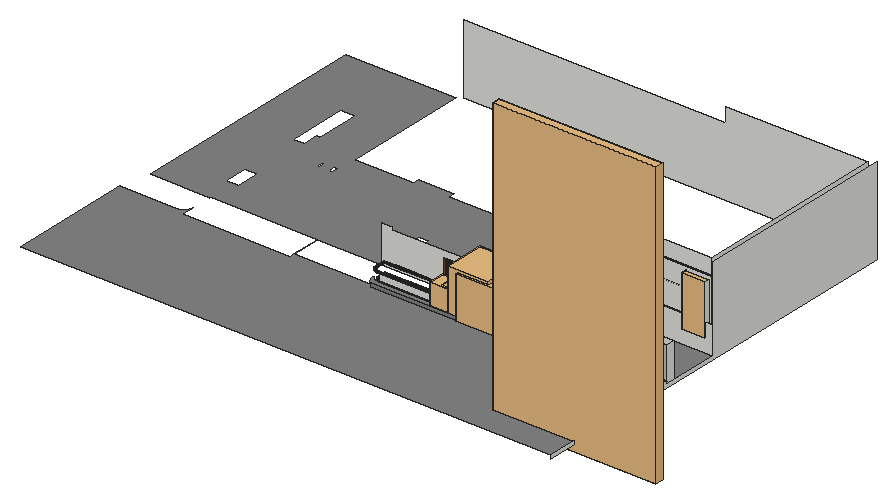
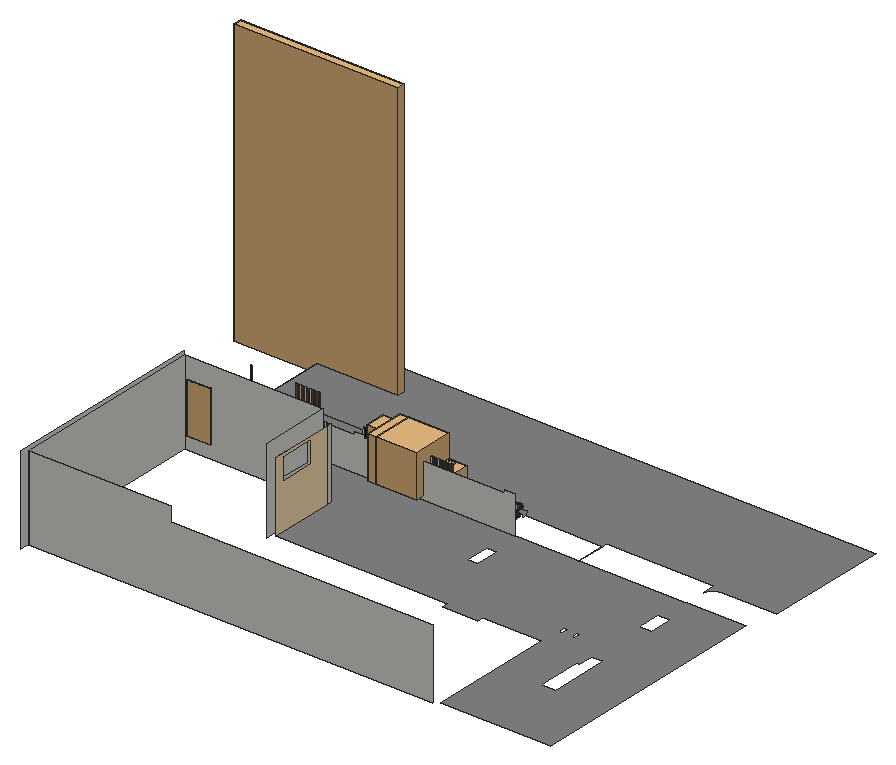
# SketchUp Ruby script. Lengths in inches.
U = 1.inch
M = Sketchup.active_model
def pt(a) = Geom::Point3d.new(a.map { |v| v * U })
def face(e, loops, mat)
  f = e.add_face(loops[0].map { |a| pt(a) })
  loops[1..].each { |l| e.add_face(l.map { |a| pt(a) }).erase! }
  f.material = f.back_material = mat if mat
  f
end
# faces: each face lists its corners as indices into pts; further lists are holes
def faces(e, pts, list, mat = nil) = list.each { |f| face(e, (f[0].is_a?(Array) ? f : [f]).map { |l| l.map { |i| pts[i] } }, mat) }
# xy, xz, yz: faces in a plane at the given z, y or x. An outline is a flat list of corners, or four numbers for a rectangle; further outlines are holes
def ring(l) = l.size == 4 ? [[l[0], l[1]], [l[2], l[1]], [l[2], l[3]], [l[0], l[3]]] : l.each_slice(2).to_a
def flat(e, list, mat, &to3) = list.each { |f| face(e, (f[0].is_a?(Array) ? f : [f]).map { |l| ring(l).map { |u, v| to3.(u, v) } }, mat) }
def xy(e, z, list, mat = nil) = flat(e, list, mat) { |x, y| [x, y, z] }
def xz(e, y, list, mat = nil) = flat(e, list, mat) { |x, z| [x, y, z] }
def yz(e, x, list, mat = nil) = flat(e, list, mat) { |y, z| [x, y, z] }
def lines(e, pts, list) = list.each { |a, b| e.add_line(pt(pts[a]), pt(pts[b])) }
# prism: a flat outline (further loops are holes) pulled along v
def prism(e, loops, v, mat = nil)
  f = face(e, loops, mat); d = Geom::Vector3d.new(v.map { |x| x * U })
  f.pushpull(f.normal.samedirection?(d) ? d.length : -d.length)
end
def box(e, o, s, mat = nil) = prism(e, [[o, [o[0] + s[0], o[1], o[2]], [o[0] + s[0], o[1] + s[1], o[2]], [o[0], o[1] + s[1], o[2]]]], [0, 0, s[2]], mat)
def at(x, y, z, deg = 0) = Geom::Transformation.translation(pt([x, y, z])) * Geom::Transformation.rotation(ORIGIN, Z_AXIS, deg.degrees)
def axes(o, x, y, z) = Geom::Transformation.new([*x, 0, *y, 0, *z, 0, *pt(o).to_a, 1])
def part(name) = M.definitions.add(name)
# library, detail: a bought-in or finely detailed component or shape, given as its bounding box
def library(name, o, s) = part(name).tap { |d| box(d.entities, o, s) }
def detail(e, o, s) = box(e.add_group.entities, o, s)
def put(e, d, t, mat = nil) = e.add_instance(d, t).tap { |i| i.material = mat if mat }
def group(e, t, mat = nil) = e.add_group.tap { |g| g.transformation = t; g.material = mat if mat }.entities
root = M.entities
M.materials.add("[0032_Moccasin]").color = [255, 228, 181]
M.materials.add("[0043_SaddleBrown]").color = [139, 69, 19]
M.materials.add("[0099_LightSteelBlue]").color = [82, 92, 104]
M.materials.add("[0131_Silver]").color = [192, 192, 192]
M.materials.add("[0136_Charcoal]").color = [35, 35, 35]
M.materials.add("[0137_Black]").color = [0, 0, 0]
M.materials.add("[Tile Grey]").color = [132, 132, 132]
M.materials.add("[Wood Veneer 01]").color = [120, 70, 37]
c1 = library("Potted plant on stand",[0,0,0],[37.88,32.09,49.42])
c2 = library("Pot+Plant",[-20.81,-17.08,-0.03],[39.86,39.43,41.33])
c3 = library("Agrupar\#180",[0,0,0],[49.83,35.16,80.22])
c4 = library("SPOT-EXTERIEUR",[0,-1.85,-3.93],[5.55,3.7,7.99])
c5 = library("A$C06767DEF\#1",[-8.3,1.21,0],[7.09,7.09,5.51])
c6 = library("door (1)",[38.93,25.48,0],[40,9.94,82.68])
c7 = library("Group\#87",[0,0,0],[185.03,8.78,321.45])
xy(root,6.6875,[[0,84.05,912.4375,84.05,912.4375,290.83,888.15,290.83,885.82,291.01,883.54,291.5625,881.37,292.46,879.37,293.68,877.59,295.2,876.0625,296.98,874.84,298.97,873.93,301.14,873.38,303.41,873.19,305.75,873.37,308.09,873.91,310.37,873.91,337.06,765.78,337.06,765.78,310.37,766.04,308.49,766.06,306.58,765.82,304.7,765.34,302.86,764.63,301.1,763.69,299.44,762.55,297.93,761.22,296.57,759.72,295.4,758.08,294.43,756.33,293.69,754.5,293.18,435,293.18,433.82,294.29,432.72,295.48,431.71,296.75,430.8,298.09,298.96,298.09,298.96,349.54,298.71,289.39,114.03,290.125,114.12,311.98,113.83,309.89,113.25,307.79,112.375,305.79,111.24,303.93,109.87,302.23,108.27,300.74,106.49,299.49,104.55,298.48,102.5,297.75,100.36,297.31,98.1875,297.16,0,297.16],[[12.79,349.54,114.27,349.54,114.27,350.28,298.96,349.54,912.4375,349.54,912.4375,431.86,798.1,431.86,798.1,432.24,795.91,432.24,795.91,431.86,720.28,431.86,720.28,432.24,713.72,432.24,713.72,433.11,711.84,433.11,711.84,432.24,705.28,432.24,705.28,433.11,703.41,433.11,703.41,432.17,696.84,432.17,696.84,433.11,694.97,433.11,694.97,432.17,688.41,432.17,688.41,433.11,686.53,433.11,686.53,432.17,679.97,432.17,679.97,433.11,677.84,433.11,677.84,432.17,671.28,432.17,671.28,433.11,669.16,433.11,669.16,432.17,666.61,432.17,666.61,431.86,660.05,431.86,660.05,551.1875,363.88,551.1875,363.88,562.07,303.76,562.07,303.76,551.1875,201.625,551.1875,201.625,768.3,12.79,768.3],[101.6875,542.92,101.6875,646.79,126.375,646.79,126.375,569.92,121.5,569.92,121.5,542.92],[101.6875,397.92,124.125,440.22],[400.76,397.92,418.84,440.22],[192.11,506.17,199.48,517.35],[171.55,506.17,177.8,517.35]]],"[Tile Grey]")
xy(root,11.9375,[[441.01,305.48,658.06,305.48,658.75,305.67,659.73,306.04,660.67,306.5,661.57,307.05,662.41,307.67,663.2,308.36,663.91,309.125,664.56,309.95,665.13,310.83,665.62,311.76,666.02,312.73,666.21,313.36,666.21,328.82,642.23,328.82,642.23,329,479.46,329,479.46,328.94,475.34,328.94,475.34,328.88,464.85,328.88,464.85,328.94,452.48,328.94,452.48,329,430.83,329,430.83,311.3,430.98,311.03,431.59,310.14,432.28,309.31,433.05,308.54,433.88,307.85,434.77,307.24,435.71,306.71,436.7,306.27,437.73,305.93,438.78,305.68,439.85,305.53]],"[0136_Charcoal]")
xy(root,11.9375,[[888.15,290.83,912.4375,290.83,912.4375,333.31,873.91,333.31,873.91,310.37,873.37,308.09,873.19,305.75,873.38,303.41,873.93,301.14,874.84,298.97,876.0625,296.98,877.59,295.2,879.37,293.68,881.37,292.46,883.54,291.5625,885.82,291.01],[435,293.18,754.5,293.18,756.33,293.69,758.08,294.43,759.72,295.4,761.22,296.57,762.55,297.93,763.69,299.44,764.63,301.1,765.34,302.86,765.82,304.7,766.06,306.58,766.04,308.49,765.78,310.37,765.78,333.31,683.875,333.31,683.875,331.81,669.83,331.81,669.83,312.81,669.42,311.49,668.89,310.22,668.25,309,667.51,307.85,666.66,306.77,665.71,305.77,664.6875,304.85,663.58,304.04,662.4,303.33,661.16,302.72,659.88,302.23,658.55,301.86,440.93,301.86,439.52,301.93,438.11,302.125,436.74,302.45,435.39,302.9,434.1,303.47,432.86,304.16,431.7,304.96,430.61,305.87,429.61,306.87,428.7,307.96,427.91,309.13,427.22,310.37,427.28,308.75,427.45,307.14,427.73,305.54,428.13,303.97,428.64,302.43,429.25,300.94,429.97,299.48,430.8,298.09,431.71,296.75,432.72,295.48,433.82,294.29]],"[Tile Grey]")
xy(root,17.45,[[765.78,337.06,873.91,337.87]])
xy(root,18.14,[[765.78,337.06,873.91,337.87]])
xy(root,26,[[[440.93,301.86,658.55,301.86,659.88,302.23,661.16,302.72,662.4,303.33,663.58,304.04,664.6875,304.85,665.71,305.77,666.66,306.77,667.51,307.85,668.25,309,668.89,310.22,669.42,311.49,669.83,312.81,669.83,333.31,669.72,333.31,669.72,332.43,666.47,332.43,666.47,333.31,665.6,333.31,665.6,332.43,662.34,332.43,662.34,333.31,661.47,333.31,661.47,332.43,658.22,332.43,658.22,333.31,657.35,333.31,657.35,332.43,654.09,332.43,654.09,333.31,653.22,333.31,653.22,332.43,649.97,332.43,649.97,333.31,649.1,333.31,649.1,332.43,645.84,332.43,645.84,333.31,644.97,333.31,644.97,332.62,641.72,332.62,641.72,333.31,640.85,333.31,640.85,332.62,637.59,332.62,637.59,333.31,636.72,333.31,636.72,332.62,633.47,332.62,633.47,333.31,632.6,333.31,632.6,332.62,629.34,332.62,629.34,333.31,628.47,333.31,628.47,332.62,625.22,332.62,625.22,333.31,624.35,333.31,624.35,332.62,621.09,332.62,621.09,333.31,620.22,333.31,620.22,332.62,616.97,332.62,616.97,333.31,616.1,333.31,616.1,332.62,612.84,332.62,612.84,333.31,611.97,333.31,611.97,332.62,608.72,332.62,608.72,333.31,607.85,333.31,607.85,332.62,604.59,332.62,604.59,333.31,603.72,333.31,603.72,332.62,600.47,332.62,600.47,333.31,599.6,333.31,599.6,332.62,596.34,332.62,596.34,333.31,595.47,333.31,595.47,332.62,592.22,332.62,592.22,333.31,591.35,333.31,591.35,332.62,588.09,332.62,588.09,333.31,587.22,333.31,587.22,332.62,583.97,332.62,583.97,333.31,583.1,333.31,583.1,332.62,579.84,332.62,579.84,333.31,578.97,333.31,578.97,332.62,575.72,332.62,575.72,333.31,574.85,333.31,574.85,332.62,571.59,332.62,571.59,333.31,570.72,333.31,570.72,332.62,567.47,332.62,567.47,333.31,566.6,333.31,566.6,332.62,563.34,332.62,563.34,333.31,562.47,333.31,562.47,332.62,559.22,332.62,559.22,333.31,558.35,333.31,558.35,332.62,555.09,332.62,555.09,333.31,554.22,333.31,554.22,332.62,550.97,332.62,550.97,333.31,550.1,333.31,550.1,332.62,546.84,332.62,546.84,333.31,545.97,333.31,545.97,332.62,542.72,332.62,542.72,333.31,541.85,333.31,541.85,332.62,538.59,332.62,538.59,333.31,537.72,333.31,537.72,332.62,534.47,332.62,534.47,333.31,533.6,333.31,533.6,332.62,530.34,332.62,530.34,333.31,529.47,333.31,529.47,332.62,526.22,332.62,526.22,333.31,525.35,333.31,525.35,332.62,522.09,332.62,522.09,333.31,521.22,333.31,521.22,332.62,517.97,332.62,517.97,333.31,517.1,333.31,517.1,332.62,513.84,332.62,513.84,333.31,512.97,333.31,512.97,332.62,509.72,332.62,509.72,333.31,508.85,333.31,508.85,332.62,505.59,332.62,505.59,333.31,504.72,333.31,504.72,332.62,501.47,332.62,501.47,333.31,500.6,333.31,500.6,332.62,497.34,332.62,497.34,333.31,496.47,333.31,496.47,332.62,493.22,332.62,493.22,333.31,492.35,333.31,492.35,332.62,489.09,332.62,489.09,333.31,488.22,333.31,488.22,332.62,484.97,332.62,484.97,333.31,484.1,333.31,484.1,332.62,480.84,332.62,480.84,333.31,479.97,333.31,479.97,332.62,476.72,332.62,476.72,333.31,475.85,333.31,475.85,332.56,472.59,332.56,472.59,333.31,471.72,333.31,471.72,332.49,468.47,332.49,468.47,333.31,467.6,333.31,467.6,332.56,464.34,332.56,464.34,333.31,463.47,333.31,463.47,332.62,460.22,332.62,460.22,333.31,459.35,333.31,459.35,332.56,456.09,332.56,456.09,333.31,455.22,333.31,455.22,332.62,451.97,332.62,451.97,333.31,451.1,333.31,451.1,332.62,447.84,332.62,447.84,333.31,446.97,333.31,446.97,332.62,443.72,332.62,443.72,333.31,442.85,333.31,442.85,332.62,439.59,332.62,439.59,333.31,438.72,333.31,438.72,332.62,435.47,332.62,435.47,333.31,434.6,333.31,434.6,332.62,431.34,332.62,431.34,333.31,430.47,333.31,430.47,332.62,427.22,332.62,427.22,310.37,427.91,309.13,428.7,307.96,429.61,306.87,430.61,305.87,431.7,304.96,432.86,304.16,434.1,303.47,435.39,302.9,436.74,302.45,438.11,302.125,439.52,301.93],[441.01,305.48,439.85,305.53,438.78,305.68,437.73,305.93,436.7,306.27,435.71,306.71,434.77,307.24,433.88,307.85,433.05,308.54,432.28,309.31,431.59,310.14,430.98,311.03,430.83,311.3,430.83,329,452.48,329,452.48,328.94,464.85,328.94,464.85,328.88,475.34,328.88,475.34,328.94,479.46,328.94,479.46,329,642.23,329,642.23,328.82,666.21,328.82,666.21,313.36,666.02,312.73,665.62,311.76,665.13,310.83,664.56,309.95,663.91,309.125,663.2,308.36,662.41,307.67,661.57,307.05,660.67,306.5,659.73,306.04,658.75,305.67,658.06,305.48]]],"[0136_Charcoal]")
xy(root,28.22,[[765.78,337.06,873.91,337.87]])
xy(root,28.91,[[765.78,337.06,873.91,337.87]])
xy(root,29.6,[[859.31,431.86,899.81,440.22]])
xy(root,38.98,[[765.78,337.06,873.91,337.87]])
xy(root,39.67,[[765.78,337.06,873.91,337.87]])
xz(root,290.83,[[888.15,6.6875,912.4375,11.9375]])
xz(root,293.18,[[435,6.6875,754.5,11.9375]],"[Tile Grey]")
xz(root,301.86,[[532.35,11.9375,533.73,26],[533.73,11.9375,535.6875,26],[535.6875,11.9375,537.0625,26],[537.0625,11.9375,539.02,26],[539.02,11.9375,540.4,26],
  [540.4,11.9375,542.36,26],[542.36,11.9375,543.73,26],[543.73,11.9375,545.69,26],[545.69,11.9375,547.07,26],[547.07,11.9375,549.03,26],
  [549.03,11.9375,550.4,26],[550.4,11.9375,552.36,26],[552.36,11.9375,553.74,26],[553.74,11.9375,555.7,26],[555.7,11.9375,557.07,26],
  [557.07,11.9375,559.03,26],[559.03,11.9375,560.41,26],[560.41,11.9375,562.37,26],[562.37,11.9375,563.74,26],[563.74,11.9375,565.7,26],
  [565.7,11.9375,567.08,26],[567.08,11.9375,569.04,26],[569.04,11.9375,570.41,26],[570.41,11.9375,572.37,26],[572.37,11.9375,573.75,26],
  [573.75,11.9375,575.71,26],[575.71,11.9375,577.08,26],[577.08,11.9375,579.04,26],[579.04,11.9375,580.42,26],[580.42,11.9375,582.375,26],
  [582.375,11.9375,583.75,26],[583.75,11.9375,585.71,26],[585.71,11.9375,587.09,26],[587.09,11.9375,589.05,26],[589.05,11.9375,590.42,26],
  [590.42,11.9375,592.38,26],[592.38,11.9375,593.75,26],[593.75,11.9375,595.72,26],[595.72,11.9375,597.09,26],[597.09,11.9375,599.05,26],
  [599.05,11.9375,600.42,26],[600.42,11.9375,602.38,26],[602.38,11.9375,603.76,26],[603.76,11.9375,605.72,26],[605.72,11.9375,607.09,26],
  [607.09,11.9375,609.05,26],[609.05,11.9375,610.43,26],[610.43,11.9375,612.39,26],[612.39,11.9375,613.76,26],[613.76,11.9375,615.72,26],
  [615.72,11.9375,617.1,26],[617.1,11.9375,619.06,26],[619.06,11.9375,620.43,26],[620.43,11.9375,622.39,26],[622.39,11.9375,623.77,26],
  [623.77,11.9375,625.73,26],[625.73,11.9375,627.1,26],[627.1,11.9375,629.0625,26],[629.0625,11.9375,630.4375,26],[630.4375,11.9375,632.4,26],
  [632.4,11.9375,633.77,26],[633.77,11.9375,635.73,26],[635.73,11.9375,637.11,26],[637.11,11.9375,639.07,26],[639.07,11.9375,640.44,26],
  [640.44,11.9375,642.4,26],[642.4,11.9375,643.78,26],[643.78,11.9375,645.74,26],[645.74,11.9375,647.11,26],[647.11,11.9375,649.07,26],
  [649.07,11.9375,650.45,26],[650.45,11.9375,652.41,26],[652.41,11.9375,653.78,26],[653.78,11.9375,655.74,26],[655.74,11.9375,657.12,26],
  [657.12,11.9375,658.55,26],[658.55,11.9375,659.08,26]],"[Wood Veneer 01]")
xz(root,305.48,[[441.01,11.9375,658.06,26]])
xz(root,328.82,[[656.84,11.9375,660.96,26],[660.96,11.9375,665.09,26],[665.09,11.9375,666.21,26]],"[0043_SaddleBrown]")
xz(root,328.82,[[642.23,11.9375,652.71,26],[652.71,11.9375,656.84,26]],"[0136_Charcoal]")
xz(root,329,[[533.09,11.9375,537.21,26],[537.21,11.9375,541.34,26],[541.34,11.9375,545.46,26],[545.46,11.9375,549.59,26],[549.59,11.9375,553.71,26],
  [553.71,11.9375,557.84,26],[557.84,11.9375,561.96,26],[561.96,11.9375,566.09,26],[566.09,11.9375,570.21,26],[570.21,11.9375,574.34,26],
  [574.34,11.9375,578.46,26],[578.46,11.9375,582.59,26],[582.59,11.9375,586.71,26],[586.71,11.9375,590.84,26],[590.84,11.9375,594.96,26],
  [594.96,11.9375,599.09,26],[599.09,11.9375,603.21,26],[603.21,11.9375,607.34,26],[607.34,11.9375,611.46,26],[611.46,11.9375,615.59,26],
  [615.59,11.9375,619.71,26],[619.71,11.9375,623.84,26],[623.84,11.9375,627.96,26],[627.96,11.9375,632.09,26],[632.09,11.9375,636.21,26],
  [636.21,11.9375,640.34,26],[640.34,11.9375,642.23,26]],"[0136_Charcoal]")
xz(root,331.81,[[669.83,11.9375,683.875,11.9375,683.875,66.6875,683.8,66.6875,683.8,70.8125,669.83,70.8125]],"[0137_Black]")
xz(root,332.43,[[645.84,26,649.1,66.6875],[649.97,26,653.22,66.6875],[654.09,26,657.35,66.6875],[658.22,26,661.47,66.6875],[662.34,26,665.6,66.6875],
  [666.47,26,669.72,66.6875]],"[Wood Veneer 01]")
xz(root,332.62,[[530.34,26,533.6,66.6875],[534.47,26,537.72,66.6875],[538.59,26,541.85,66.6875],[542.72,26,545.97,66.6875],[546.84,26,550.1,66.6875],
  [550.97,26,554.22,66.6875],[555.09,26,558.35,66.6875],[559.22,26,562.47,66.6875],[563.34,26,566.6,66.6875],[567.47,26,570.72,66.6875],
  [571.59,26,574.85,66.6875],[575.72,26,578.97,66.6875],[579.84,26,583.1,66.6875],[583.97,26,587.22,66.6875],[588.09,26,591.35,66.6875],
  [592.22,26,595.47,66.6875],[596.34,26,599.6,66.6875],[600.47,26,603.72,66.6875],[604.59,26,607.85,66.6875],[608.72,26,611.97,66.6875],
  [612.84,26,616.1,66.6875],[616.97,26,620.22,66.6875],[621.09,26,624.35,66.6875],[625.22,26,628.47,66.6875],[629.34,26,632.6,66.6875],
  [633.47,26,636.72,66.6875],[637.59,26,640.85,66.6875],[641.72,26,644.97,66.6875]],"[Wood Veneer 01]")
xz(root,333.31,[[669.72,26,669.83,66.6875]])
xz(root,333.31,[[683.875,11.9375,765.78,11.9375,765.78,49.75,873.91,49.75,873.91,11.9375,912.4375,11.9375,912.4375,66.6875,683.875,66.6875]],"[0131_Silver]")
xz(root,333.31,[[533.6,26,534.47,66.6875],[537.72,26,538.59,66.6875],[541.85,26,542.72,66.6875],[545.97,26,546.84,66.6875],[550.1,26,550.97,66.6875],
  [554.22,26,555.09,66.6875],[558.35,26,559.22,66.6875],[562.47,26,563.34,66.6875],[566.6,26,567.47,66.6875],[570.72,26,571.59,66.6875],
  [574.85,26,575.72,66.6875],[578.97,26,579.84,66.6875],[583.1,26,583.97,66.6875],[587.22,26,588.09,66.6875],[591.35,26,592.22,66.6875],
  [595.47,26,596.34,66.6875],[599.6,26,600.47,66.6875],[603.72,26,604.59,66.6875],[607.85,26,608.72,66.6875],[611.97,26,612.84,66.6875],
  [616.1,26,616.97,66.6875],[620.22,26,621.09,66.6875],[624.35,26,625.22,66.6875],[628.47,26,629.34,66.6875],[632.6,26,633.47,66.6875],
  [636.72,26,637.59,66.6875],[640.85,26,641.72,66.6875],[644.97,26,645.84,66.6875],[649.1,26,649.97,66.6875],[653.22,26,654.09,66.6875],
  [657.35,26,658.22,66.6875],[661.47,26,662.34,66.6875],[665.6,26,666.47,66.6875]],"[Wood Veneer 01]")
xz(root,337.06,[[765.78,6.6875,873.91,17.45],[765.78,18.14,873.91,28.22],[765.78,28.91,873.91,38.98],[765.78,39.67,873.91,49.75]],"[0099_LightSteelBlue]")
xz(root,337.87,[[765.78,17.45,873.91,18.14],[765.78,28.22,873.91,28.91],[765.78,38.98,873.91,39.67]])
xz(root,349.54,[[408.98,6.6875,408.98,70.8125,427.22,70.8125,427.22,66.6875,669.83,66.6875,669.83,70.8125,683.8,70.8125,683.8,66.6875,912.4375,66.6875,912.4375,6.6875]])
xz(root,431.86,[[720.28,6.6875,795.91,54.15],[798.1,6.6875,912.4375,6.6875,912.4375,54.15,899.81,54.15,899.81,29.6,859.31,29.6,859.31,54.15,798.1,54.15]])
xz(root,431.86,[[660.05,6.6875,666.61,126.6875]],"[Wood Veneer 01]")
xz(root,432.17,[[666.61,6.6875,669.16,126.6875],[671.28,6.6875,677.84,126.6875],[679.97,6.6875,686.53,169.25],[688.41,6.6875,694.97,169.25],[696.84,6.6875,703.41,169.25]],"[Wood Veneer 01]")
xz(root,432.24,[[795.91,6.6875,798.1,6.6875,798.1,54.15,859.31,54.15,859.31,55.72,798.1,55.72,798.1,95.09,859.31,95.09,859.31,96.15,798.1,96.15,798.1,128.97,912.4375,128.97,912.4375,130.53,798.1,130.53,798.1,169.25,795.91,169.25,795.91,130.53,720.28,130.53,720.28,128.97,795.91,128.97,795.91,96.15,720.28,96.15,720.28,95.09,795.91,95.09,795.91,55.72,720.28,55.72,720.28,54.15,795.91,54.15]],"[0136_Charcoal]")
xz(root,432.24,[[705.28,6.6875,711.84,169.25],[713.72,6.6875,720.28,169.25]],"[Wood Veneer 01]")
xz(root,433.11,[[669.16,6.6875,671.28,126.6875],[677.84,6.6875,679.97,6.6875,679.97,169.25,678.11,169.25,678.11,126.6875,677.84,126.6875],[686.53,6.6875,688.41,169.25],[694.97,6.6875,696.84,169.25],[703.41,6.6875,705.28,169.25],
  [711.84,6.6875,713.72,169.25]])
xz(root,440.22,[[[666.61,6.6875,904.08,151.4375],[859.31,29.6,899.81,115.98]]])
xz(root,775.6875,[[209.98,6.6875,904.08,6.6875,904.08,151.4375,660.05,151.4375,660.05,126.6875,209.98,126.6875]])
yz(root,533.6,[[332.62,26,333.31,66.6875]],"[Wood Veneer 01]")
yz(root,534.47,[[332.62,26,333.31,66.6875]])
yz(root,537.72,[[332.62,26,333.31,66.6875]],"[Wood Veneer 01]")
yz(root,538.59,[[332.62,26,333.31,66.6875]])
yz(root,541.85,[[332.62,26,333.31,66.6875]])
yz(root,542.72,[[332.62,26,333.31,66.6875]])
yz(root,545.97,[[332.62,26,333.31,66.6875]])
yz(root,546.84,[[332.62,26,333.31,66.6875]])
yz(root,550.1,[[332.62,26,333.31,66.6875]])
yz(root,550.97,[[332.62,26,333.31,66.6875]])
yz(root,554.22,[[332.62,26,333.31,66.6875]])
yz(root,555.09,[[332.62,26,333.31,66.6875]])
yz(root,558.35,[[332.62,26,333.31,66.6875]])
yz(root,559.22,[[332.62,26,333.31,66.6875]])
yz(root,562.47,[[332.62,26,333.31,66.6875]])
yz(root,563.34,[[332.62,26,333.31,66.6875]])
yz(root,566.6,[[332.62,26,333.31,66.6875]])
yz(root,567.47,[[332.62,26,333.31,66.6875]])
yz(root,570.72,[[332.62,26,333.31,66.6875]])
yz(root,571.59,[[332.62,26,333.31,66.6875]])
yz(root,574.85,[[332.62,26,333.31,66.6875]])
yz(root,575.72,[[332.62,26,333.31,66.6875]])
yz(root,578.97,[[332.62,26,333.31,66.6875]])
yz(root,579.84,[[332.62,26,333.31,66.6875]])
yz(root,583.1,[[332.62,26,333.31,66.6875]])
yz(root,583.97,[[332.62,26,333.31,66.6875]])
yz(root,587.22,[[332.62,26,333.31,66.6875]])
yz(root,588.09,[[332.62,26,333.31,66.6875]])
yz(root,591.35,[[332.62,26,333.31,66.6875]])
yz(root,592.22,[[332.62,26,333.31,66.6875]])
yz(root,595.47,[[332.62,26,333.31,66.6875]])
yz(root,596.34,[[332.62,26,333.31,66.6875]])
yz(root,599.6,[[332.62,26,333.31,66.6875]])
yz(root,600.47,[[332.62,26,333.31,66.6875]])
yz(root,603.72,[[332.62,26,333.31,66.6875]])
yz(root,604.59,[[332.62,26,333.31,66.6875]])
yz(root,607.85,[[332.62,26,333.31,66.6875]],"[Wood Veneer 01]")
yz(root,608.72,[[332.62,26,333.31,66.6875]])
yz(root,611.97,[[332.62,26,333.31,66.6875]],"[Wood Veneer 01]")
yz(root,612.84,[[332.62,26,333.31,66.6875]])
yz(root,616.1,[[332.62,26,333.31,66.6875]],"[Wood Veneer 01]")
yz(root,616.97,[[332.62,26,333.31,66.6875]])
yz(root,620.22,[[332.62,26,333.31,66.6875]],"[Wood Veneer 01]")
yz(root,621.09,[[332.62,26,333.31,66.6875]])
yz(root,624.35,[[332.62,26,333.31,66.6875]],"[Wood Veneer 01]")
yz(root,625.22,[[332.62,26,333.31,66.6875]])
yz(root,628.47,[[332.62,26,333.31,66.6875]],"[Wood Veneer 01]")
yz(root,629.34,[[332.62,26,333.31,66.6875]])
yz(root,632.6,[[332.62,26,333.31,66.6875]],"[Wood Veneer 01]")
yz(root,633.47,[[332.62,26,333.31,66.6875]])
yz(root,636.72,[[332.62,26,333.31,66.6875]],"[Wood Veneer 01]")
yz(root,637.59,[[332.62,26,333.31,66.6875]],"[Wood Veneer 01]")
yz(root,640.85,[[332.62,26,333.31,66.6875]],"[Wood Veneer 01]")
yz(root,641.72,[[332.62,26,333.31,66.6875]],"[Wood Veneer 01]")
yz(root,642.23,[[328.82,11.9375,329,26]])
yz(root,644.97,[[332.62,26,333.31,66.6875]])
yz(root,645.84,[[332.43,26,333.31,66.6875]],"[Wood Veneer 01]")
yz(root,649.1,[[332.43,26,333.31,66.6875]])
yz(root,649.97,[[332.43,26,333.31,66.6875]],"[Wood Veneer 01]")
yz(root,653.22,[[332.43,26,333.31,66.6875]],"[Wood Veneer 01]")
yz(root,654.09,[[332.43,26,333.31,66.6875]])
yz(root,657.35,[[332.43,26,333.31,66.6875]],"[Wood Veneer 01]")
yz(root,658.22,[[332.43,26,333.31,66.6875]])
yz(root,660.05,[[431.86,6.6875,440.22,126.6875]])
yz(root,660.05,[[[440.22,6.6875,551.1875,126.6875],[474.23,84.24,536.02,122.43]]],"[0032_Moccasin]")
yz(root,661.47,[[332.43,26,333.31,66.6875]])
yz(root,662.34,[[332.43,26,333.31,66.6875]])
yz(root,665.6,[[332.43,26,333.31,66.6875]])
yz(root,666.21,[[313.36,11.9375,328.82,26]],"[0043_SaddleBrown]")
yz(root,666.47,[[332.43,26,333.31,66.6875]])
yz(root,666.61,[[431.86,6.6875,432.17,126.6875],[[440.22,6.6875,562.07,151.4375],[474.23,84.24,536.02,122.43]]])
yz(root,669.16,[[432.17,6.6875,433.11,126.6875]])
yz(root,669.72,[[332.43,26,333.31,66.6875]])
yz(root,669.83,[[331.81,26,333.31,66.6875]])
yz(root,669.83,[[312.81,11.9375,331.81,26]],"[Wood Veneer 01]")
yz(root,671.28,[[432.17,6.6875,433.11,126.6875]])
yz(root,677.84,[[432.17,6.6875,433.11,126.6875]])
yz(root,679.97,[[432.17,6.6875,433.11,169.25]])
yz(root,683.875,[[331.81,11.9375,333.31,66.6875]])
yz(root,686.53,[[432.17,6.6875,433.11,169.25]])
yz(root,688.41,[[432.17,6.6875,433.11,169.25]])
yz(root,694.97,[[432.17,6.6875,433.11,169.25]])
yz(root,696.84,[[432.17,6.6875,433.11,169.25]])
yz(root,703.41,[[432.17,6.6875,433.11,169.25]])
yz(root,705.28,[[432.24,6.6875,433.11,169.25]])
yz(root,711.84,[[432.24,6.6875,433.11,169.25]])
yz(root,713.72,[[432.24,6.6875,433.11,169.25]])
yz(root,720.28,[[431.86,6.6875,432.24,54.15]])
yz(root,765.78,[[333.31,11.9375,337.06,11.9375,337.06,17.45,337.87,17.45,337.87,18.14,337.06,18.14,337.06,28.22,337.87,28.22,337.87,28.91,337.06,28.91,337.06,38.98,337.87,38.98,337.87,39.67,337.06,39.67,337.06,49.75,333.31,49.75]])
yz(root,765.78,[[310.37,6.6875,337.06,11.9375]],"[Tile Grey]")
yz(root,795.91,[[431.86,6.6875,432.24,8],[431.86,8,432.24,54.15]])
yz(root,798.1,[[431.86,6.6875,432.24,8],[431.86,8,432.24,54.15]])
yz(root,859.31,[[431.86,29.6,440.22,29.6,440.22,115.98,431.86,115.98,431.86,96.15,432.24,96.15,432.24,95.09,431.86,95.09,431.86,55.72,432.24,55.72,432.24,54.15,431.86,54.15]])
yz(root,873.91,[[310.37,6.6875,337.06,11.9375],[333.31,11.9375,333.31,49.75,337.06,49.75,337.06,39.67,337.87,39.67,337.87,38.98,337.06,38.98,337.06,28.91,337.87,28.91,337.87,28.22,337.06,28.22,337.06,18.14,337.87,18.14,337.87,17.45,337.06,17.45,337.06,11.9375]])
yz(root,899.81,[[431.86,29.6,431.86,54.15,432.24,54.15,432.24,55.72,431.86,55.72,431.86,95.09,432.24,95.09,432.24,96.15,431.86,96.15,431.86,115.98,440.22,115.98,440.22,29.6]])
yz(root,904.08,[[440.22,6.6875,775.6875,151.4375]])
yz(root,912.4375,[[84.05,0,784.05,0,784.05,151.4375,431.86,151.4375,431.86,130.53,432.24,130.53,432.24,128.97,431.86,128.97,431.86,96.15,432.24,96.15,432.24,95.09,431.86,95.09,431.86,55.72,432.24,55.72,432.24,54.15,431.86,54.15,431.86,6.6875,333.31,6.6875,333.31,11.9375,290.83,11.9375,290.83,6.6875,84.05,6.6875],[333.31,6.6875,349.54,66.6875]])
p = [[885.82,291.01,6.6875],[888.15,290.83,6.6875],[888.15,290.83,11.9375],[885.82,291.01,11.9375],[883.54,291.5625,6.6875],[883.54,291.5625,11.9375],
  [881.37,292.46,6.6875],[881.37,292.46,11.9375],[879.37,293.68,6.6875],[879.37,293.68,11.9375],[754.5,293.18,6.6875],[756.33,293.69,6.6875],
  [756.33,293.69,11.9375],[754.5,293.18,11.9375],[758.08,294.43,6.6875],[758.08,294.43,11.9375],[877.59,295.2,6.6875],[877.59,295.2,11.9375],
  [759.72,295.4,6.6875],[759.72,295.4,11.9375],[876.0625,296.98,6.6875],[876.0625,296.98,11.9375],[761.22,296.57,6.6875],[761.22,296.57,11.9375],
  [762.55,297.93,6.6875],[762.55,297.93,11.9375],[874.84,298.97,6.6875],[874.84,298.97,11.9375],[763.69,299.44,6.6875],[763.69,299.44,11.9375],
  [873.93,301.14,6.6875],[873.93,301.14,11.9375],[764.63,301.1,6.6875],[764.63,301.1,11.9375],[765.34,302.86,6.6875],[765.34,302.86,11.9375],
  [873.38,303.41,6.6875],[873.38,303.41,11.9375],[765.82,304.7,6.6875],[765.82,304.7,11.9375],[873.19,305.75,6.6875],[873.19,305.75,11.9375],
  [766.06,306.58,6.6875],[766.06,306.58,11.9375],[873.37,308.09,6.6875],[873.37,308.09,11.9375],[766.04,308.49,6.6875],[766.04,308.49,11.9375],
  [873.91,310.37,6.6875],[873.91,310.37,11.9375],[765.78,310.37,6.6875],[765.78,310.37,11.9375],[658.55,301.86,11.9375],[659.88,302.23,11.9375],
  [659.88,302.23,26],[658.55,301.86,26],[661.16,302.72,11.9375],[661.16,302.72,26],[662.4,303.33,11.9375],[662.4,303.33,26],
  [663.58,304.04,11.9375],[663.58,304.04,26],[664.6875,304.85,11.9375],[664.6875,304.85,26],[665.71,305.77,11.9375],[665.71,305.77,26],
  [658.75,305.67,11.9375],[658.06,305.48,11.9375],[658.06,305.48,26],[658.75,305.67,26],[659.73,306.04,11.9375],[659.73,306.04,26],
  [666.66,306.77,11.9375],[666.66,306.77,26],[660.67,306.5,11.9375],[660.67,306.5,26],[661.57,307.05,11.9375],[661.57,307.05,26],
  [667.51,307.85,11.9375],[667.51,307.85,26],[662.41,307.67,11.9375],[662.41,307.67,26],[663.2,308.36,11.9375],[663.2,308.36,26],
  [668.25,309,11.9375],[668.25,309,26],[663.91,309.125,11.9375],[663.91,309.125,26],[668.89,310.22,11.9375],[668.89,310.22,26],
  [664.56,309.95,11.9375],[664.56,309.95,26],[665.13,310.83,11.9375],[665.13,310.83,26],[669.42,311.49,11.9375],[669.42,311.49,26],
  [665.62,311.76,11.9375],[665.62,311.76,26],[669.83,312.81,11.9375],[669.83,312.81,26],[666.02,312.73,11.9375],[666.02,312.73,26],
  [666.21,313.36,11.9375],[666.21,313.36,26],[662.59,433.11,126.6875],[662.59,433.11,6.6875]]
faces(root,p,[[0,1,2,3],[4,0,3,5],[6,4,5,7],[8,6,7,9],[16,8,9,17],[20,16,17,21],[26,20,21,27],[30,26,27,31],
  [36,30,31,37],[40,36,37,41],[44,40,41,45],[48,44,45,49],[66,67,68,69],[70,66,69,71],[74,70,71,75],[76,74,75,77],
  [80,76,77,81],[82,80,81,83],[86,82,83,87],[90,86,87,91],[92,90,91,93],[96,92,93,97],[100,96,97,101],[102,100,101,103]])
faces(root,p,[[10,11,12,13],[11,14,15,12],[14,18,19,15],[18,22,23,19],[22,24,25,23],[24,28,29,25],[28,32,33,29],[32,34,35,33],
  [34,38,39,35],[38,42,43,39],[42,46,47,43],[46,50,51,47]],"[Tile Grey]")
faces(root,p,[[52,53,54,55],[53,56,57,54],[56,58,59,57],[58,60,61,59],[60,62,63,61],[62,64,65,63],[64,72,73,65],[72,78,79,73],
  [78,84,85,79],[84,88,89,85],[88,94,95,89],[94,98,99,95]],"[Wood Veneer 01]")
lines(root,p,[[104,105]])
put(root,c1,axes([534.88,295.93,4.2],[0.87,0,0],[0,0.87,0],[0,0,0.87]))
put(root,c1,axes([551.43,300.05,4.07],[0.87,0,0],[0,0.87,0],[0,0,0.87]),"[0136_Charcoal]")
put(root,c1,axes([570.49,300.05,4.07],[0.87,0,0],[0,0.87,0],[0,0,0.87]))
put(root,c2,axes([604.01,323.25,12],[1.76,0,0],[0,1.76,0],[0,0,1.76]),"[Wood Veneer 01]")
put(root,c2,axes([622.34,318.25,8.45],[1.76,0,0],[0,1.76,0],[0,0,1.76]),"[Wood Veneer 01]")
put(root,c3,at(624.55,301.38,-1.375),"[Wood Veneer 01]")
put(root,c4,at(720.97,324.33,1.92,-90))
put(root,c5,axes([822.11,333.35,48.58],[0.36702,0,0],[0,0.44707,0],[0,0,0.28]))
put(root,c6,axes([820.38,406.375,29.6],[1,0,0],[0,1,0],[0,0,1.04473]))
put(root,c7,axes([773.5625,132.72,-9.11],[1.52,0,0],[0,1.52,0],[0,0,1.52]))
